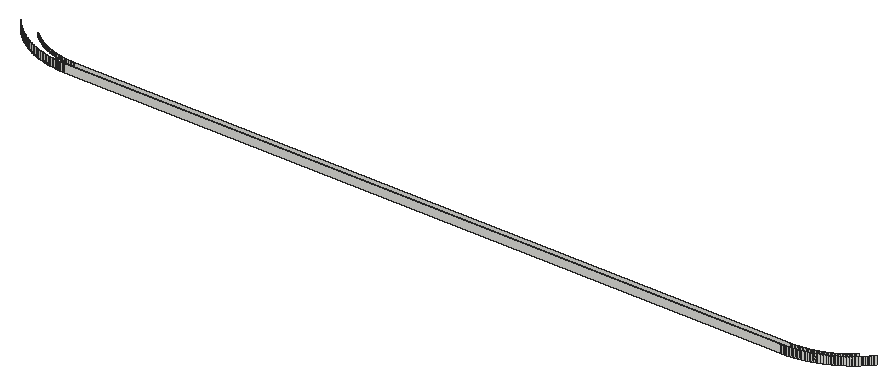
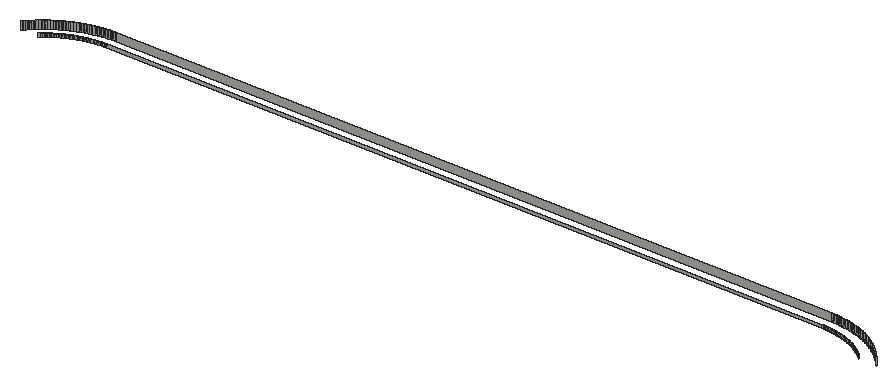
# SketchUp Ruby script. Lengths in inches.
U = 1.inch
M = Sketchup.active_model
def pt(a) = Geom::Point3d.new(a.map { |v| v * U })
def face(e, loops, mat)
  f = e.add_face(loops[0].map { |a| pt(a) })
  loops[1..].each { |l| e.add_face(l.map { |a| pt(a) }).erase! }
  f.material = f.back_material = mat if mat
  f
end
# faces: each face lists its corners as indices into pts; further lists are holes
def faces(e, pts, list, mat = nil) = list.each { |f| face(e, (f[0].is_a?(Array) ? f : [f]).map { |l| l.map { |i| pts[i] } }, mat) }
# xy, xz, yz: faces in a plane at the given z, y or x. An outline is a flat list of corners, or four numbers for a rectangle; further outlines are holes
def ring(l) = l.size == 4 ? [[l[0], l[1]], [l[2], l[1]], [l[2], l[3]], [l[0], l[3]]] : l.each_slice(2).to_a
def flat(e, list, mat, &to3) = list.each { |f| face(e, (f[0].is_a?(Array) ? f : [f]).map { |l| ring(l).map { |u, v| to3.(u, v) } }, mat) }
def xy(e, z, list, mat = nil) = flat(e, list, mat) { |x, y| [x, y, z] }
def xz(e, y, list, mat = nil) = flat(e, list, mat) { |x, z| [x, y, z] }
def yz(e, x, list, mat = nil) = flat(e, list, mat) { |y, z| [x, y, z] }
def lines(e, pts, list) = list.each { |a, b| e.add_line(pt(pts[a]), pt(pts[b])) }
# prism: a flat outline (further loops are holes) pulled along v
def prism(e, loops, v, mat = nil)
  f = face(e, loops, mat); d = Geom::Vector3d.new(v.map { |x| x * U })
  f.pushpull(f.normal.samedirection?(d) ? d.length : -d.length)
end
def box(e, o, s, mat = nil) = prism(e, [[o, [o[0] + s[0], o[1], o[2]], [o[0] + s[0], o[1] + s[1], o[2]], [o[0], o[1] + s[1], o[2]]]], [0, 0, s[2]], mat)
def at(x, y, z, deg = 0) = Geom::Transformation.translation(pt([x, y, z])) * Geom::Transformation.rotation(ORIGIN, Z_AXIS, deg.degrees)
def axes(o, x, y, z) = Geom::Transformation.new([*x, 0, *y, 0, *z, 0, *pt(o).to_a, 1])
def part(name) = M.definitions.add(name)
# library, detail: a bought-in or finely detailed component or shape, given as its bounding box
def library(name, o, s) = part(name).tap { |d| box(d.entities, o, s) }
def detail(e, o, s) = box(e.add_group.entities, o, s)
def put(e, d, t, mat = nil) = e.add_instance(d, t).tap { |i| i.material = mat if mat }
def group(e, t, mat = nil) = e.add_group.tap { |g| g.transformation = t; g.material = mat if mat }.entities
root = M.entities
xz(root,204,[[38.61,347,39,349.5],[39,347,270,349.5],[270,347,270.39,349.5]])
xz(root,208,[[38.66,347,39,348],[39,347,270,348],[270,347,270.34,348]])
p = [[37.43,204.04,349.5],[37.04,204.0625,349.5],[37.04,204.0625,347],[37.43,204.04,347],[37.82,204.02,349.5],[37.82,204.02,347],
  [38.21,204.01,349.5],[38.21,204.01,347],[38.61,204,349.5],[38.61,204,347],[270.79,204.01,349.5],[270.39,204,349.5],
  [270.39,204,347],[270.79,204.01,347],[271.18,204.02,349.5],[271.18,204.02,347],[271.57,204.04,349.5],[271.57,204.04,347],
  [271.96,204.0625,349.5],[271.96,204.0625,347],[36.25,204.125,349.5],[35.86,204.16,349.5],[35.86,204.16,347],[36.25,204.125,347],
  [36.65,204.09,349.5],[36.65,204.09,347],[272.35,204.09,349.5],[272.35,204.09,347],[272.75,204.125,349.5],[272.75,204.125,347],
  [273.14,204.16,349.5],[273.14,204.16,347],[35.47,204.21,349.5],[35.08,204.26,349.5],[35.08,204.26,347],[35.47,204.21,347],
  [273.53,204.21,349.5],[273.53,204.21,347],[273.92,204.26,349.5],[273.92,204.26,347],[34.7,204.31,349.5],[34.31,204.37,349.5],
  [34.31,204.37,347],[34.7,204.31,347],[274.3,204.31,349.5],[274.3,204.31,347],[274.69,204.37,349.5],[274.69,204.37,347],
  [33.92,204.43,349.5],[33.53,204.5,349.5],[33.53,204.5,347],[33.92,204.43,347],[275.08,204.43,349.5],[275.08,204.43,347],
  [275.47,204.5,349.5],[275.47,204.5,347],[33.15,204.58,349.5],[33.15,204.58,347],[275.85,204.58,349.5],[275.85,204.58,347],
  [32.76,204.66,349.5],[32.76,204.66,347],[276.24,204.66,349.5],[276.24,204.66,347],[32.38,204.74,349.5],[32,204.83,349.5],
  [32,204.83,347],[32.38,204.74,347],[276.62,204.74,349.5],[276.62,204.74,347],[277,204.83,349.5],[277,204.83,347],
  [31.62,204.92,349.5],[31.62,204.92,347],[277.38,204.92,349.5],[277.38,204.92,347],[31.24,205.02,349.5],[31.24,205.02,347],
  [277.76,205.02,349.5],[277.76,205.02,347],[30.86,205.125,349.5],[30.86,205.125,347],[278.14,205.125,349.5],[278.14,205.125,347],
  [30.48,205.24,349.5],[30.48,205.24,347],[278.52,205.24,349.5],[278.52,205.24,347],[30.1,205.35,349.5],[30.1,205.35,347],
  [278.9,205.35,349.5],[278.9,205.35,347],[29.73,205.47,349.5],[29.73,205.47,347],[279.27,205.47,349.5],[279.27,205.47,347],
  [29.36,205.59,349.5],[29.36,205.59,347],[279.64,205.59,349.5],[279.64,205.59,347],[28.99,205.72,349.5],[28.99,205.72,347],
  [280.01,205.72,349.5],[280.01,205.72,347],[28.62,205.85,349.5],[28.62,205.85,347],[280.38,205.85,349.5],[280.38,205.85,347],
  [28.25,205.99,349.5],[28.25,205.99,347],[280.75,205.99,349.5],[280.75,205.99,347],[27.88,206.14,349.5],[27.88,206.14,347],
  [281.12,206.14,349.5],[281.12,206.14,347],[27.52,206.28,349.5],[27.52,206.28,347],[281.48,206.28,349.5],[281.48,206.28,347],
  [27.16,206.4375,349.5],[27.16,206.4375,347],[281.84,206.4375,349.5],[281.84,206.4375,347],[26.8,206.59,349.5],[26.8,206.59,347],
  [282.2,206.59,349.5],[282.2,206.59,347],[26.44,206.76,349.5],[26.44,206.76,347],[282.56,206.76,349.5],[282.56,206.76,347],
  [26.08,206.92,349.5],[26.08,206.92,347],[282.92,206.92,349.5],[282.92,206.92,347],[25.73,207.09,349.5],[25.73,207.09,347],
  [283.27,207.09,349.5],[283.27,207.09,347],[25.38,207.27,349.5],[25.38,207.27,347],[283.62,207.27,349.5],[283.62,207.27,347],
  [25.03,207.45,349.5],[25.03,207.45,347],[283.97,207.45,349.5],[283.97,207.45,347],[24.69,207.64,349.5],[24.69,207.64,347],
  [284.31,207.64,349.5],[284.31,207.64,347],[24.34,207.83,349.5],[24.34,207.83,347],[284.66,207.83,349.5],[284.66,207.83,347],
  [24,208.02,349.5],[24,208.02,347],[285,208.02,349.5],[285,208.02,347],[23.66,208.22,349.5],[23.66,208.22,347],
  [37.64,208.04,347],[37.3,208.06,347],[37.3,208.06,348],[37.64,208.04,348],[37.98,208.02,347],[37.98,208.02,348],
  [38.32,208.01,347],[38.32,208.01,348],[38.66,208,347],[38.66,208,348],[270.68,208.01,347],[270.34,208,347],
  [270.34,208,348],[270.68,208.01,348],[271.02,208.02,347],[271.02,208.02,348],[271.36,208.04,347],[271.36,208.04,348],
  [271.7,208.06,347],[271.7,208.06,348],[285.34,208.22,349.5],[285.34,208.22,347],[36.28,208.14,347],[35.94,208.18,347],
  [35.94,208.18,348],[36.28,208.14,348],[36.62,208.11,347],[36.62,208.11,348],[36.96,208.08,347],[36.96,208.08,348],
  [272.04,208.08,347],[272.04,208.08,348],[272.38,208.11,347],[272.38,208.11,348],[272.72,208.14,347],[272.72,208.14,348],
  [273.06,208.18,347],[273.06,208.18,348],[23.33,208.42,349.5],[23.33,208.42,347],[35.61,208.22,347],[35.27,208.27,347],
  [35.27,208.27,348],[35.61,208.22,348],[273.39,208.22,347],[273.39,208.22,348],[273.73,208.27,347],[273.73,208.27,348],
  [285.67,208.42,349.5],[285.67,208.42,347],[34.93,208.32,347],[34.6,208.375,347],[34.6,208.375,348],[34.93,208.32,348],
  [274.07,208.32,347],[274.07,208.32,348],[274.4,208.375,347],[274.4,208.375,348],[22.99,208.63,349.5],[22.99,208.63,347],
  [34.26,208.44,347],[33.93,208.5,347],[33.93,208.5,348],[34.26,208.44,348],[274.74,208.44,347],[274.74,208.44,348],
  [275.07,208.5,347],[275.07,208.5,348],[286.01,208.63,349.5],[286.01,208.63,347],[33.59,208.57,347],[33.59,208.57,348],
  [275.41,208.57,347],[275.41,208.57,348],[22.66,208.84,349.5],[22.66,208.84,347],[33.26,208.64,347],[32.93,208.72,347],
  [32.93,208.72,348],[33.26,208.64,348],[275.74,208.64,347],[275.74,208.64,348],[276.07,208.72,347],[276.07,208.72,348],
  [286.34,208.84,349.5],[286.34,208.84,347],[32.6,208.8,347],[32.6,208.8,348],[276.4,208.8,347],[276.4,208.8,348],
  [22.33,209.06,349.5],[22.33,209.06,347],[32.27,208.89,347],[32.27,208.89,348],[276.73,208.89,347],[276.73,208.89,348],
  [286.67,209.06,349.5],[286.67,209.06,347],[31.94,208.98,347],[31.94,208.98,348],[277.06,208.98,347],[277.06,208.98,348],
  [31.62,209.07,347],[31.62,209.07,348],[277.38,209.07,347],[277.38,209.07,348],[22.01,209.28,349.5],[22.01,209.28,347],
  [31.29,209.17,347],[31.29,209.17,348],[277.71,209.17,347],[277.71,209.17,348],[286.99,209.28,349.5],[286.99,209.28,347],
  [30.97,209.27,347],[30.97,209.27,348],[278.03,209.27,347],[278.03,209.27,348],[21.6875,209.5,349.5],[21.6875,209.5,347],
  [30.64,209.38,347],[30.64,209.38,348],[278.36,209.38,347],[278.36,209.38,348],[287.3125,209.5,349.5],[287.3125,209.5,347],
  [30.32,209.49,347],[30.32,209.49,348],[278.68,209.49,347],[278.68,209.49,348],[21.37,209.73,349.5],[21.37,209.73,347],
  [30,209.61,347],[30,209.61,348],[279,209.61,347],[279,209.61,348],[287.63,209.73,349.5],[287.63,209.73,347],
  [29.68,209.73,347],[29.68,209.73,348],[279.32,209.73,347],[279.32,209.73,348],[21.05,209.96,349.5],[21.05,209.96,347],
  [29.37,209.85,347],[29.37,209.85,348],[279.63,209.85,347],[279.63,209.85,348],[287.95,209.96,349.5],[287.95,209.96,347],
  [29.05,209.98,347],[29.05,209.98,348],[279.95,209.98,347],[279.95,209.98,348],[20.74,210.2,349.5],[20.74,210.2,347],
  [28.74,210.11,347],[28.74,210.11,348],[280.26,210.11,347],[280.26,210.11,348],[288.26,210.2,349.5],[288.26,210.2,347],
  [28.42,210.25,347],[28.42,210.25,348],[280.58,210.25,347],[280.58,210.25,348],[20.43,210.44,349.5],[20.43,210.44,347],
  [28.11,210.39,347],[28.11,210.39,348],[280.89,210.39,347],[280.89,210.39,348],[288.57,210.44,349.5],[288.57,210.44,347],
  [20.12,210.6875,349.5],[20.12,210.6875,347],[27.81,210.53,347],[27.81,210.53,348],[281.19,210.53,347],[281.19,210.53,348],
  [288.88,210.6875,349.5],[288.88,210.6875,347],[27.5,210.68,347],[27.5,210.68,348],[281.5,210.68,347],[281.5,210.68,348],
  [19.82,210.93,349.5],[19.82,210.93,347],[27.2,210.83,347],[27.2,210.83,348],[281.8,210.83,347],[281.8,210.83,348],
  [289.18,210.93,349.5],[289.18,210.93,347],[26.89,210.99,347],[26.89,210.99,348],[282.11,210.99,347],[282.11,210.99,348],
  [19.52,211.1875,349.5],[19.52,211.1875,347],[289.48,211.1875,349.5],[289.48,211.1875,347],[26.59,211.15,347],[26.59,211.15,348],
  [282.41,211.15,347],[282.41,211.15,348],[19.22,211.44,349.5],[19.22,211.44,347],[26.3,211.32,347],[26.3,211.32,348],
  [282.7,211.32,347],[282.7,211.32,348],[289.78,211.44,349.5],[289.78,211.44,347],[26,211.48,347],[26,211.48,348],
  [283,211.48,347],[283,211.48,348],[18.93,211.71,349.5],[18.93,211.71,347],[290.07,211.71,349.5],[290.07,211.71,347],
  [25.71,211.66,347],[25.71,211.66,348],[283.29,211.66,347],[283.29,211.66,348],[18.64,211.97,349.5],[18.64,211.97,347],
  [25.42,211.83,347],[25.42,211.83,348],[283.58,211.83,347],[283.58,211.83,348],[290.36,211.97,349.5],[290.36,211.97,347],
  [25.125,212.01,347],[25.125,212.01,348],[283.875,212.01,347],[283.875,212.01,348],[18.35,212.24,349.5],[18.35,212.24,347],
  [24.84,212.19,347],[24.84,212.19,348],[284.16,212.19,347],[284.16,212.19,348],[290.65,212.24,349.5],[290.65,212.24,347],
  [18.07,212.51,349.5],[18.07,212.51,347],[24.56,212.38,347],[24.56,212.38,348],[284.44,212.38,347],[284.44,212.38,348],
  [290.93,212.51,349.5],[290.93,212.51,347],[24.27,212.57,347],[24.27,212.57,348],[284.73,212.57,347],[284.73,212.57,348],
  [17.79,212.79,349.5],[17.79,212.79,347],[291.21,212.79,349.5],[291.21,212.79,347],[23.99,212.77,347],[23.99,212.77,348],
  [285.01,212.77,347],[285.01,212.77,348],[17.51,213.07,349.5],[17.51,213.07,347],[23.72,212.97,347],[23.72,212.97,348],
  [285.28,212.97,347],[285.28,212.97,348],[291.49,213.07,349.5],[291.49,213.07,347],[23.44,213.17,347],[23.44,213.17,348],
  [285.56,213.17,347],[285.56,213.17,348],[17.24,213.35,349.5],[17.24,213.35,347],[291.76,213.35,349.5],[291.76,213.35,347],
  [23.17,213.37,347],[23.17,213.37,348],[285.83,213.37,347],[285.83,213.37,348],[16.97,213.64,349.5],[16.97,213.64,347],
  [292.03,213.64,349.5],[292.03,213.64,347],[22.9,213.58,347],[22.9,213.58,348],[286.1,213.58,347],[286.1,213.58,348],
  [16.71,213.93,349.5],[16.71,213.93,347],[22.64,213.79,347],[22.64,213.79,348],[286.36,213.79,347],[286.36,213.79,348],
  [292.29,213.93,349.5],[292.29,213.93,347],[22.375,214.01,347],[22.375,214.01,348],[286.625,214.01,347],[286.625,214.01,348],
  [16.44,214.22,349.5],[16.44,214.22,347],[292.56,214.22,349.5],[292.56,214.22,347],[22.11,214.23,347],[22.11,214.23,348],
  [286.89,214.23,347],[286.89,214.23,348],[16.1875,214.52,349.5],[16.1875,214.52,347],[21.86,214.45,347],[21.86,214.45,348],
  [287.14,214.45,347],[287.14,214.45,348],[292.8125,214.52,349.5],[292.8125,214.52,347]]
faces(root,p,[[0,1,2,3],[4,0,3,5],[6,4,5,7],[8,6,7,9],[10,11,12,13],[14,10,13,15],[16,14,15,17],[18,16,17,19],
  [20,21,22,23],[24,20,23,25],[1,24,25,2],[26,18,19,27],[28,26,27,29],[30,28,29,31],[32,33,34,35],[21,32,35,22],
  [36,30,31,37],[38,36,37,39],[40,41,42,43],[33,40,43,34],[44,38,39,45],[46,44,45,47],[48,49,50,51],[41,48,51,42],
  [52,46,47,53],[54,52,53,55],[49,56,57,50],[58,54,55,59],[56,60,61,57],[62,58,59,63],[64,65,66,67],[60,64,67,61],
  [68,62,63,69],[70,68,69,71],[65,72,73,66],[74,70,71,75],[72,76,77,73],[78,74,75,79],[76,80,81,77],[82,78,79,83],
  [80,84,85,81],[86,82,83,87],[84,88,89,85],[90,86,87,91],[88,92,93,89],[94,90,91,95],[92,96,97,93],[98,94,95,99],
  [96,100,101,97],[102,98,99,103],[100,104,105,101],[106,102,103,107],[104,108,109,105],[110,106,107,111],[108,112,113,109],[114,110,111,115],
  [112,116,117,113],[118,114,115,119],[116,120,121,117],[122,118,119,123],[120,124,125,121],[126,122,123,127],[124,128,129,125],[130,126,127,131],
  [128,132,133,129],[134,130,131,135],[132,136,137,133],[138,134,135,139],[136,140,141,137],[142,138,139,143],[140,144,145,141],[146,142,143,147],
  [144,148,149,145],[150,146,147,151],[148,152,153,149],[154,150,151,155],[152,156,157,153],[158,154,155,159],[156,160,161,157],[162,163,164,165],
  [166,162,165,167],[168,166,167,169],[170,168,169,171],[172,173,174,175],[176,172,175,177],[178,176,177,179],[180,178,179,181],[182,158,159,183],
  [184,185,186,187],[188,184,187,189],[190,188,189,191],[163,190,191,164],[192,180,181,193],[194,192,193,195],[196,194,195,197],[198,196,197,199],
  [160,200,201,161],[202,203,204,205],[185,202,205,186],[206,198,199,207],[208,206,207,209],[210,182,183,211],[212,213,214,215],[203,212,215,204],
  [216,208,209,217],[218,216,217,219],[200,220,221,201],[222,223,224,225],[213,222,225,214],[226,218,219,227],[228,226,227,229],[230,210,211,231],
  [223,232,233,224],[234,228,229,235],[220,236,237,221],[238,239,240,241],[232,238,241,233],[242,234,235,243],[244,242,243,245],[246,230,231,247],
  [239,248,249,240],[250,244,245,251],[236,252,253,237],[248,254,255,249],[256,250,251,257],[258,246,247,259],[254,260,261,255],[262,256,257,263],
  [260,264,265,261],[266,262,263,267],[252,268,269,253],[264,270,271,265],[272,266,267,273],[274,258,259,275],[270,276,277,271],[278,272,273,279],
  [268,280,281,269],[276,282,283,277],[284,278,279,285],[286,274,275,287],[282,288,289,283],[290,284,285,291],[280,292,293,281],[288,294,295,289],
  [296,290,291,297],[298,286,287,299],[294,300,301,295],[302,296,297,303],[292,304,305,293],[300,306,307,301],[308,302,303,309],[310,298,299,311],
  [306,312,313,307],[314,308,309,315],[304,316,317,305],[312,318,319,313],[320,314,315,321],[322,310,311,323],[318,324,325,319],[326,320,321,327],
  [316,328,329,317],[324,330,331,325],[332,326,327,333],[334,322,323,335],[328,336,337,329],[330,338,339,331],[340,332,333,341],[342,334,335,343],
  [338,344,345,339],[346,340,341,347],[336,348,349,337],[344,350,351,345],[352,346,347,353],[354,342,343,355],[350,356,357,351],[358,352,353,359],
  [348,360,361,349],[362,354,355,363],[356,364,365,357],[366,358,359,367],[360,368,369,361],[364,370,371,365],[372,366,367,373],[374,362,363,375],
  [370,376,377,371],[378,372,373,379],[368,380,381,369],[382,374,375,383],[376,384,385,377],[386,378,379,387],[380,388,389,381],[384,390,391,385],
  [392,386,387,393],[394,382,383,395],[390,396,397,391],[398,392,393,399],[388,400,401,389],[396,402,403,397],[404,398,399,405],[406,394,395,407],
  [400,408,409,401],[402,410,411,403],[412,404,405,413],[414,406,407,415],[410,416,417,411],[418,412,413,419],[408,420,421,409],[422,414,415,423],
  [416,424,425,417],[426,418,419,427],[420,428,429,421],[424,430,431,425],[432,426,427,433],[434,422,423,435],[430,436,437,431],[438,432,433,439],
  [428,440,441,429],[442,434,435,443],[436,444,445,437],[446,438,439,447],[440,448,449,441],[450,442,443,451],[444,452,453,445],[454,446,447,455],
  [448,456,457,449],[452,458,459,453],[460,454,455,461],[462,450,451,463],[458,464,465,459],[466,460,461,467],[456,468,469,457],[470,462,463,471],
  [464,472,473,465],[474,466,467,475],[468,476,477,469],[472,478,479,473],[480,474,475,481],[482,470,471,483]])
